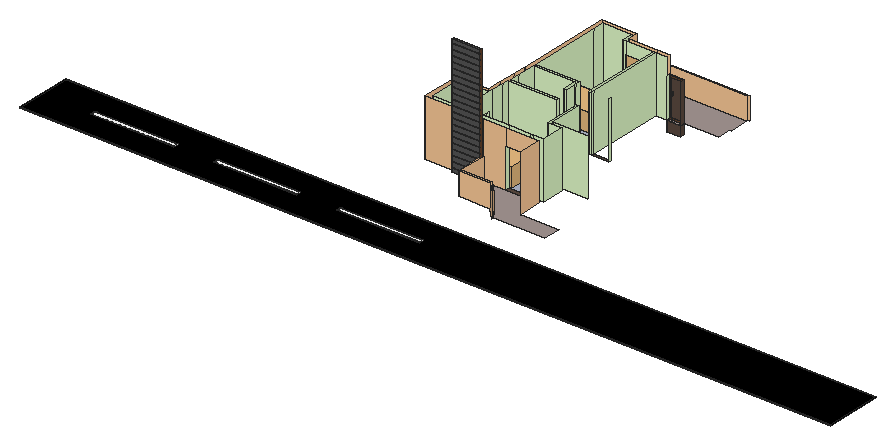
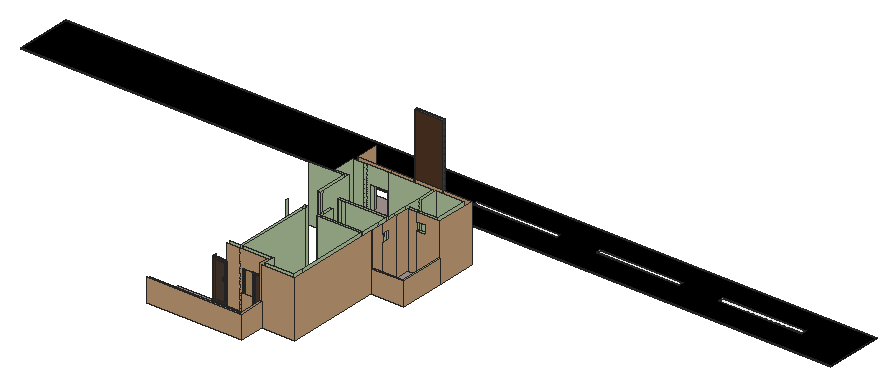
# SketchUp Ruby script. Lengths in inches.
U = 1.inch
M = Sketchup.active_model
def pt(a) = Geom::Point3d.new(a.map { |v| v * U })
def face(e, loops, mat)
  f = e.add_face(loops[0].map { |a| pt(a) })
  loops[1..].each { |l| e.add_face(l.map { |a| pt(a) }).erase! }
  f.material = f.back_material = mat if mat
  f
end
# faces: each face lists its corners as indices into pts; further lists are holes
def faces(e, pts, list, mat = nil) = list.each { |f| face(e, (f[0].is_a?(Array) ? f : [f]).map { |l| l.map { |i| pts[i] } }, mat) }
# xy, xz, yz: faces in a plane at the given z, y or x. An outline is a flat list of corners, or four numbers for a rectangle; further outlines are holes
def ring(l) = l.size == 4 ? [[l[0], l[1]], [l[2], l[1]], [l[2], l[3]], [l[0], l[3]]] : l.each_slice(2).to_a
def flat(e, list, mat, &to3) = list.each { |f| face(e, (f[0].is_a?(Array) ? f : [f]).map { |l| ring(l).map { |u, v| to3.(u, v) } }, mat) }
def xy(e, z, list, mat = nil) = flat(e, list, mat) { |x, y| [x, y, z] }
def xz(e, y, list, mat = nil) = flat(e, list, mat) { |x, z| [x, y, z] }
def yz(e, x, list, mat = nil) = flat(e, list, mat) { |y, z| [x, y, z] }
def lines(e, pts, list) = list.each { |a, b| e.add_line(pt(pts[a]), pt(pts[b])) }
# prism: a flat outline (further loops are holes) pulled along v
def prism(e, loops, v, mat = nil)
  f = face(e, loops, mat); d = Geom::Vector3d.new(v.map { |x| x * U })
  f.pushpull(f.normal.samedirection?(d) ? d.length : -d.length)
end
def box(e, o, s, mat = nil) = prism(e, [[o, [o[0] + s[0], o[1], o[2]], [o[0] + s[0], o[1] + s[1], o[2]], [o[0], o[1] + s[1], o[2]]]], [0, 0, s[2]], mat)
def at(x, y, z, deg = 0) = Geom::Transformation.translation(pt([x, y, z])) * Geom::Transformation.rotation(ORIGIN, Z_AXIS, deg.degrees)
def axes(o, x, y, z) = Geom::Transformation.new([*x, 0, *y, 0, *z, 0, *pt(o).to_a, 1])
def part(name) = M.definitions.add(name)
# library, detail: a bought-in or finely detailed component or shape, given as its bounding box
def library(name, o, s) = part(name).tap { |d| box(d.entities, o, s) }
def detail(e, o, s) = box(e.add_group.entities, o, s)
def put(e, d, t, mat = nil) = e.add_instance(d, t).tap { |i| i.material = mat if mat }
def group(e, t, mat = nil) = e.add_group.tap { |g| g.transformation = t; g.material = mat if mat }.entities
root = M.entities
M.materials.add("C02_Golden_Beige").color = [255, 205, 155]
M.materials.add("F01_Seafoam_Drift").color = [229, 255, 204]
M.materials.add("M00_Soft_Cloud").color = [255, 255, 255]
M.materials.add("M01_Silver_Fog").color = [224, 224, 224]
M.materials.add("M03_Pewter_Shine").color = [168, 168, 168]
M.materials.add("M04_Stone_Frost").color = [142, 142, 142]
M.materials.add("M06_Steel_Smoke").color = [86, 86, 86]
M.materials.add("M09_Shadow_Night").color = [0, 0, 0]
M.materials.add("Marble_03_1K").color = [175, 182, 201]
M.materials.add("Marble_06_1K").color = [165, 150, 147]
M.materials.add("Marble_20_1K").color = [172, 173, 182]
M.materials.add("Metal_06_1K").color = [238, 236, 231]
M.materials.add("Wood_Floor_12_1K").color = [92, 75, 65]
M.materials.add("Wood_Veneer_15_1K").color = [103, 69, 45]
c1 = part("Group\#73")
box(c1.entities,[0,0,0],[176.75,20.5625,0.9])
c2 = library("Toilet 005",[-7.26,-21.97,0],[14.52,21.97,16.93])
c3 = library("Marcel Lift Bed Queen",[-31.83,-34.39,0],[63.66,83.19,38.98])
c4 = part("Group\#9")
xy(c4.entities,0,[[0,0,40.3125,19.1]])
xy(c4.entities,16,[[8.1875,0.77,29.4,18.21]])
xy(c4.entities,21.0625,[[0,0,40.3125,19.1]])
xy(c4.entities,25,[[[0,0,40.3125,19.1],[8.1875,0.77,29.4,18.21]]])
xy(c4.entities,25.5,[[[0,0,40.3125,19.1],[8.1875,0.77,29.4,18.21]]],"M09_Shadow_Night")
xz(c4.entities,-0.1875,[[20.17,22.3,20.39,22.33,20.61,22.42,20.79,22.56,20.93,22.74,21.01,22.95,21.04,23.18,21.01,23.4,20.93,23.61,20.79,23.8,20.61,23.93,20.39,24.02,20.17,24.05,19.94,24.02,19.73,23.93,19.55,23.8,19.41,23.61,19.32,23.4,19.29,23.18,19.32,22.95,19.41,22.74,19.55,22.56,19.73,22.42,19.94,22.33]],"M03_Pewter_Shine")
xz(c4.entities,0,[[19.56,0,20.76,21.0625],[0,25,40.3125,25.5]],"M09_Shadow_Night")
xz(c4.entities,0,[[0,0,19.56,21.0625],[20.76,0,40.3125,21.0625],[[0,21.0625,40.3125,25],[20.17,22.3,19.94,22.33,19.73,22.42,19.55,22.56,19.41,22.74,19.32,22.95,19.29,23.18,19.32,23.4,19.41,23.61,19.55,23.8,19.73,23.93,19.94,24.02,20.17,24.05,20.39,24.02,20.61,23.93,20.79,23.8,20.93,23.61,21.01,23.4,21.04,23.18,21.01,22.95,20.93,22.74,20.79,22.56,20.61,22.42,20.39,22.33]]],"Wood_Veneer_15_1K")
xz(c4.entities,0.77,[[8.1875,16,29.4,25]])
xz(c4.entities,0.77,[[8.1875,25,29.4,25.5]],"M04_Stone_Frost")
xz(c4.entities,18.21,[[8.1875,16,29.4,25],[8.1875,25,29.4,25.5]])
xz(c4.entities,19.1,[[0,25,40.3125,25.5]],"M09_Shadow_Night")
xz(c4.entities,19.1,[[0,0,40.3125,21.0625],[0,21.0625,40.3125,25]],"Wood_Veneer_15_1K")
yz(c4.entities,0,[[0,25,19.1,25.5]],"M09_Shadow_Night")
yz(c4.entities,0,[[0,0,19.1,21.0625],[0,21.0625,19.1,25]],"Wood_Veneer_15_1K")
yz(c4.entities,8.1875,[[0.77,16,18.21,25]])
yz(c4.entities,8.1875,[[0.77,25,18.21,25.5]],"M04_Stone_Frost")
yz(c4.entities,29.4,[[0.77,16,18.21,25]])
yz(c4.entities,29.4,[[0.77,25,18.21,25.5]],"M04_Stone_Frost")
yz(c4.entities,40.3125,[[0,25,19.1,25.5]],"M09_Shadow_Night")
yz(c4.entities,40.3125,[[0,0,19.1,21.0625],[0,21.0625,19.1,25]],"Wood_Veneer_15_1K")
p = [[19.73,0,22.42],[19.94,0,22.33],[19.94,-0.1875,22.33],[19.73,-0.1875,22.42],[20.17,0,22.3],[20.17,-0.1875,22.3],
  [20.39,0,22.33],[20.39,-0.1875,22.33],[20.61,0,22.42],[20.61,-0.1875,22.42],[19.55,0,22.56],[19.55,-0.1875,22.56],
  [20.79,0,22.56],[20.79,-0.1875,22.56],[19.41,0,22.74],[19.41,-0.1875,22.74],[20.93,0,22.74],[20.93,-0.1875,22.74],
  [19.32,0,22.95],[19.32,-0.1875,22.95],[21.01,0,22.95],[21.01,-0.1875,22.95],[19.29,0,23.18],[19.29,-0.1875,23.18],
  [21.04,0,23.18],[21.04,-0.1875,23.18],[19.32,0,23.4],[19.32,-0.1875,23.4],[21.01,0,23.4],[21.01,-0.1875,23.4],
  [19.41,0,23.61],[19.41,-0.1875,23.61],[20.93,0,23.61],[20.93,-0.1875,23.61],[19.55,0,23.8],[19.55,-0.1875,23.8],
  [20.79,0,23.8],[20.79,-0.1875,23.8],[19.73,0,23.93],[19.73,-0.1875,23.93],[20.61,0,23.93],[20.61,-0.1875,23.93],
  [19.94,0,24.02],[19.94,-0.1875,24.02],[20.39,0,24.02],[20.39,-0.1875,24.02],[20.17,0,24.05],[20.17,-0.1875,24.05]]
faces(c4.entities,p,[[0,1,2,3],[1,4,5,2],[4,6,7,5],[6,8,9,7],[10,0,3,11],[8,12,13,9],[14,10,11,15],[12,16,17,13],
  [18,14,15,19],[16,20,21,17],[22,18,19,23],[20,24,25,21],[26,22,23,27],[24,28,29,25],[30,26,27,31],[28,32,33,29],
  [34,30,31,35],[32,36,37,33],[38,34,35,39],[36,40,41,37],[42,38,39,43],[40,44,45,41],[46,42,43,47],[44,46,47,45]],"M03_Pewter_Shine")
g1 = group(c4.entities,at(16.89,0,11.23),"M01_Silver_Fog")
box(g1,[0,-0.1875,0],[1.125,0.1875,4],"M03_Pewter_Shine")
g2 = group(c4.entities,at(22.02,0,11.23),"M01_Silver_Fog")
box(g2,[0,-0.1875,0],[1.125,0.1875,4],"M03_Pewter_Shine")
c5 = part("Group\#25")
xy(c5.entities,0,[[0,-3,30,0]],"Wood_Veneer_15_1K")
xy(c5.entities,3,[[3,-2.25,27,0]],"Wood_Floor_12_1K")
xy(c5.entities,3,[[3,-3,27,-2.25]],"Wood_Veneer_15_1K")
xy(c5.entities,81,[[3,-2.25,27,0]],"Wood_Floor_12_1K")
xy(c5.entities,81,[[3,-3,27,-2.25]],"Wood_Veneer_15_1K")
xy(c5.entities,84,[[0,-3,30,0]],"Wood_Veneer_15_1K")
xz(c5.entities,-3,[[[0,0,30,84],[3,3,27,81]]],"Wood_Veneer_15_1K")
xz(c5.entities,-2.25,[[3,3,27,81]],"Wood_Floor_12_1K")
xz(c5.entities,0,[[[0,0,30,84],[3,3,27,81]]],"Wood_Veneer_15_1K")
yz(c5.entities,0,[[-3,0,0,84]],"Wood_Veneer_15_1K")
yz(c5.entities,3,[[-2.25,3,0,81]],"Wood_Floor_12_1K")
yz(c5.entities,3,[[-3,3,-2.25,81]],"Wood_Veneer_15_1K")
yz(c5.entities,27,[[-2.25,3,0,81]],"Wood_Floor_12_1K")
yz(c5.entities,27,[[-3,3,-2.25,81]],"Wood_Veneer_15_1K")
yz(c5.entities,30,[[-3,0,0,84]],"Wood_Veneer_15_1K")
g3 = group(c5.entities,at(22.875,-2.25,50.47),"Metal_06_1K")
xy(g3,-5.5625,[[0,-0.48,1.25,0]],"Metal_06_1K")
xy(g3,-4.9375,[[0,-1.375,1.25,-0.48]],"Metal_06_1K")
xy(g3,-4.6875,[[0,-1.125,1.25,0]],"Metal_06_1K")
xy(g3,-4.6875,[[0,-1.375,1.25,-1.125]],"Wood_Veneer_15_1K")
xy(g3,0,[[0,-1.125,1.25,-0.5],[0,-0.5,1.25,0]],"Metal_06_1K")
xy(g3,0.25,[[0,-1.375,1.25,-1.125],[0,-1.125,1.25,-0.5]],"Metal_06_1K")
xy(g3,0.25,[[0,-0.5,1.25,0]],"Wood_Veneer_15_1K")
xy(g3,1.25,[[0,-0.5,1.25,0]],"Metal_06_1K")
xz(g3,-1.375,[[0,-4.9375,1.25,-4.6875],[0,-4.6875,1.25,0.25]],"Metal_06_1K")
xz(g3,-1.125,[[0,-4.6875,1.25,0],[0,0,1.25,0.25]],"Metal_06_1K")
xz(g3,-0.5,[[0,0.25,1.25,1.25]],"Metal_06_1K")
xz(g3,-0.5,[[0,0,1.25,0.25]],"Wood_Veneer_15_1K")
xz(g3,-0.48,[[0,-5.5625,1.25,-4.9375]],"Metal_06_1K")
xz(g3,0,[[0,0.25,1.25,1.25]],"Metal_06_1K")
xz(g3,0,[[0,-5.5625,1.25,-4.6875],[0,0,1.25,0.25]],"Wood_Veneer_15_1K")
yz(g3,0,[[-0.48,-5.5625,-0.48,-4.9375,-1.375,-4.9375,-1.375,-4.6875,0,-4.6875,0,-5.5625],[-1.375,-4.6875,-1.125,0.25],[-1.125,0,-0.5,0.25],[-0.5,0,0,0.25],[-0.5,0.25,0,1.25]],"Metal_06_1K")
yz(g3,1.25,[[-0.48,-5.5625,0,-5.5625,0,-4.6875,-1.375,-4.6875,-1.375,-4.9375,-0.48,-4.9375],[-1.375,-4.6875,-1.125,0.25],[-1.125,0,-0.5,0.25],[-0.5,0,0,0.25],[-0.5,0.25,0,1.25]],"Metal_06_1K")
c6 = library("Group\#19",[0,0,0],[54,1.88,94.04])
box(root,[1542.8125,897.17,20.5625],[9,18.21,0.4375],"Wood_Floor_12_1K")
xy(root,-0.6875,[[1705.83,1117.375,1735.83,1126.375]],"Wood_Floor_12_1K")
xy(root,11.375,[[1619.1875,1117.375,1649.1875,1126.375]],"F01_Seafoam_Drift")
xy(root,22,[[1548.8125,772.375,1689.8125,889.375],[1689.8125,772.375,1719.8125,819.6875],[1645.8125,951.6875,1677.8125,951.6875,1677.8125,1117.375,1551.8125,1117.375,1551.8125,961.375,1645.8125,961.375]],"Marble_03_1K")
xy(root,22,[[1688.52,678.6875,1797.92,678.6875,1797.92,714.6875,1716.8125,714.6875,1716.8125,763.375,1599.1,763.375,1599.1,703.375,1664.03,703.375],[1482.8125,772.375,1542.8125,841.375],[1477.8125,847.375,1542.8125,941.875],[1551.8125,1117.375,1613.1875,1141.375],[1705.83,1117.375,1735.83,1126.375],
  [1619.1875,1126.375,1809.8125,1126.375,1809.8125,1156.375,1812.8125,1156.375,1812.8125,1198.375,1619.1875,1198.375]],"Marble_06_1K")
xy(root,22,[[1551.8125,895.375,1639.8125,955.375]],"Marble_20_1K")
xy(root,22,[[1645.59,763.375,1681.59,772.375],[1542.8125,811.375,1548.8125,841.375],[1653.8125,889.375,1689.8125,895.375],[1639.8125,895.375,1645.8125,925.375],[1645.8125,945.6875,1677.8125,951.6875],
  [1683.8125,945.6875,1719.8125,951.6875],[1649.1875,1117.375,1651.0625,1126.375]],"Wood_Floor_12_1K")
xz(root,700.375,[[1596.1,21,1662.78,70]],"C02_Golden_Beige")
xz(root,703.375,[[1599.1,22,1664.03,70]],"C02_Golden_Beige")
xz(root,763.375,[[1473.8125,21,1596.1,142],[1599.1,22,1645.59,142],[1681.59,22,1716.8125,22,1716.8125,142,1645.59,142,1645.59,106,1681.59,106]],"C02_Golden_Beige")
xz(root,772.375,[[1482.8125,22,1542.8125,142],[1548.8125,22,1645.59,142],[1681.59,22,1681.59,106,1645.59,106,1645.59,142,1689.8125,142,1689.8125,22],[1689.8125,22,1695.8125,142],[1695.8125,22,1719.8125,142]],"F01_Seafoam_Drift")
xz(root,811.375,[[1542.8125,22,1548.8125,106]],"F01_Seafoam_Drift")
xz(root,819.6875,[[1689.8125,22,1719.8125,142]],"F01_Seafoam_Drift")
xz(root,825.6875,[[1695.8125,22,1770.625,142]],"F01_Seafoam_Drift")
xz(root,841.375,[[1482.8125,22,1523.47,22,1523.47,106,1504.12,106,1504.12,124,1523.47,124,1523.47,142,1482.8125,142],[1523.47,22,1542.8125,142],[1542.8125,22,1548.8125,106]],"F01_Seafoam_Drift")
xz(root,847.375,[[1477.8125,22,1477.8125,142,1523.47,142,1523.47,124,1504.12,124,1504.12,106,1523.47,106,1523.47,22],[1523.47,22,1542.8125,142]],"C02_Golden_Beige")
xz(root,889.375,[[1548.8125,22,1653.8125,142]],"F01_Seafoam_Drift")
xz(root,895.375,[[1551.8125,22,1639.8125,142],[1639.8125,22,1645.8125,142],[1645.8125,22,1653.8125,142],[1689.8125,22,1695.8125,142]],"F01_Seafoam_Drift")
xz(root,925.375,[[1639.8125,22,1645.8125,142]],"F01_Seafoam_Drift")
xz(root,941.875,[[1477.8125,22,1542.8125,70]],"C02_Golden_Beige")
xz(root,944.875,[[1473.8125,21,1542.8125,70]],"C02_Golden_Beige")
xz(root,945.6875,[[1677.8125,22,1683.8125,142]],"F01_Seafoam_Drift")
xz(root,955.375,[[1551.8125,22,1639.8125,142]],"F01_Seafoam_Drift")
xz(root,961.375,[[1551.8125,22,1645.8125,142]],"F01_Seafoam_Drift")
xz(root,1117.375,[[1619.1875,11.375,1649.1875,22],[1613.1875,22,1619.1875,142],[1673.1875,22,1677.8125,22,1677.8125,142,1619.1875,142,1619.1875,106,1673.1875,106],[1683.8125,22,1705.83,142]],"F01_Seafoam_Drift")
xz(root,1117.375,[[1705.83,-0.6875,1735.83,22],[1649.1875,22,1651.0625,106],[1651.0625,22,1673.1875,58]],"Wood_Floor_12_1K")
xz(root,1126.375,[[1673.1875,22,1673.1875,106,1619.1875,106,1619.1875,142,1677.8125,142,1677.8125,22],[1649.1875,22,1651.0625,106],[1651.0625,22,1673.1875,58],[1677.8125,22,1705.83,142]],"C02_Golden_Beige")
xz(root,1126.375,[[1619.1875,11.375,1649.1875,22]],"F01_Seafoam_Drift")
xz(root,1126.375,[[1705.83,-0.6875,1735.83,22]],"Wood_Floor_12_1K")
xz(root,1141.375,[[1551.8125,22,1613.1875,142]],"F01_Seafoam_Drift")
xz(root,1147.375,[[1542.8125,21,1613.1875,142]],"C02_Golden_Beige")
xz(root,1198.375,[[1619.1875,22,1812.8125,70]],"C02_Golden_Beige")
xz(root,1201.375,[[1613.1875,21,1815.8125,70]],"C02_Golden_Beige")
yz(root,1473.8125,[[763.375,21,847.375,142],[847.375,21,944.875,70]],"C02_Golden_Beige")
yz(root,1477.8125,[[847.375,22,941.875,70]],"F01_Seafoam_Drift")
yz(root,1482.8125,[[772.375,22,841.375,142]],"F01_Seafoam_Drift")
yz(root,1542.8125,[[944.875,21,1147.375,142],[847.375,22,877.375,142],[877.375,22,877.375,142,915.375,142,915.375,124,897.17,124,897.17,106,915.375,106,915.375,22],[915.375,22,941.875,142]],"C02_Golden_Beige")
yz(root,1542.8125,[[772.375,22,811.375,142]],"F01_Seafoam_Drift")
yz(root,1548.8125,[[772.375,22,811.375,142],[841.375,22,847.375,22,847.375,142,811.375,142,811.375,106,841.375,106],[847.375,22,877.375,142],[877.375,22,889.375,142]],"F01_Seafoam_Drift")
yz(root,1551.8125,[[895.375,22,915.375,22,915.375,106,897.17,106,897.17,124,915.375,124,915.375,142,895.375,142],[915.375,22,955.375,142],[961.375,22,1117.375,142],[1117.375,22,1141.375,142]],"F01_Seafoam_Drift")
yz(root,1596.1,[[700.375,21,763.375,70]],"C02_Golden_Beige")
yz(root,1599.1,[[703.375,22,763.375,70]],"C02_Golden_Beige")
yz(root,1613.1875,[[1147.375,21,1201.375,70]],"C02_Golden_Beige")
yz(root,1613.1875,[[1117.375,22,1141.375,142]],"F01_Seafoam_Drift")
yz(root,1619.1875,[[1126.375,22,1147.375,142],[1147.375,22,1198.375,70]],"C02_Golden_Beige")
yz(root,1619.1875,[[1117.375,11.375,1126.375,106]],"F01_Seafoam_Drift")
yz(root,1639.8125,[[925.375,22,955.375,142]],"F01_Seafoam_Drift")
yz(root,1645.59,[[763.375,22,772.375,106]],"F01_Seafoam_Drift")
yz(root,1645.8125,[[925.375,22,945.6875,142],[945.6875,22,951.6875,142],[951.6875,22,961.375,142]],"F01_Seafoam_Drift")
yz(root,1649.1875,[[1117.375,11.375,1126.375,22]],"F01_Seafoam_Drift")
yz(root,1649.1875,[[1117.375,22,1126.375,106]],"Wood_Floor_12_1K")
yz(root,1651.0625,[[1117.375,22,1126.375,58]],"Wood_Floor_12_1K")
yz(root,1653.8125,[[889.375,22,895.375,142]],"F01_Seafoam_Drift")
yz(root,1677.8125,[[945.6875,22,951.6875,142],[951.6875,22,1117.375,142]],"F01_Seafoam_Drift")
yz(root,1681.59,[[763.375,22,772.375,106]],"F01_Seafoam_Drift")
yz(root,1683.8125,[[945.6875,22,951.6875,142],[951.6875,22,1117.375,142]],"F01_Seafoam_Drift")
yz(root,1689.8125,[[819.6875,22,889.375,142],[889.375,22,895.375,142]],"F01_Seafoam_Drift")
yz(root,1695.8125,[[825.6875,22,895.375,142]],"F01_Seafoam_Drift")
yz(root,1705.83,[[1117.375,22,1126.375,106]],"F01_Seafoam_Drift")
yz(root,1705.83,[[1117.375,-0.6875,1126.375,22]],"Wood_Floor_12_1K")
yz(root,1716.8125,[[714.6875,22,763.375,142]],"C02_Golden_Beige")
yz(root,1719.8125,[[772.375,22,819.6875,142],[945.6875,22,951.6875,142]],"F01_Seafoam_Drift")
yz(root,1735.83,[[1117.375,-0.6875,1126.375,22],[1117.375,22,1126.375,106]],"Wood_Floor_12_1K")
p = [[1662.78,700.375,21],[1687.27,675.6875,21],[1687.27,675.6875,70],[1662.78,700.375,70],[1688.52,678.6875,22],[1664.03,703.375,22],
  [1664.03,703.375,70],[1688.52,678.6875,70],[1735.83,1117.375,21],[1735.83,1126.375,21],[1711.83,1117.375,21],[1711.83,1126.375,21]]
faces(root,p,[[0,1,2,3],[4,5,6,7]],"C02_Golden_Beige")
lines(root,p,[[8,9],[8,10],[11,9],[11,10]])
put(root,c1,axes([921.69,563.94,1],[1,0,0],[0,0.43638,0],[0,0,1]),"M00_Soft_Cloud")
put(root,c1,axes([1183.63,563.94,1],[1,0,0],[0,0.43638,0],[0,0,1]),"M00_Soft_Cloud")
put(root,c2,at(1483.51,804.98,22,90),"M01_Silver_Fog")
put(root,c1,axes([1445.57,563.94,1],[1,0,0],[0,0.43638,0],[0,0,1]),"M00_Soft_Cloud")
put(root,c2,at(1553.39,922.33,22,90),"M01_Silver_Fog")
g4 = group(root,at(1473.8125,763,21),"Marble_03_1K")
xy(g4,0,[[62.46,-5.8125,62.4375,0.1875,122.28,0.37,122.3,-5.63]],"Wood_Veneer_15_1K")
xy(g4,254,[[62.46,-5.8125,122.3,-5.63,122.28,0.37,62.4375,0.1875]],"M06_Steel_Smoke")
p = [[62.4375,0.1875,254],[62.4375,0.1875,0],[62.46,-5.8125,0],[62.46,-5.8125,7.89],[62.46,-5.8125,9.48],[62.46,-5.8125,19.79],
  [62.46,-5.8125,21.38],[62.46,-5.8125,31.68],[62.46,-5.8125,33.28],[62.46,-5.8125,43.57],[62.46,-5.8125,45.18],[62.46,-5.8125,55.46],
  [62.46,-5.8125,57.08],[62.46,-5.8125,67.36],[62.46,-5.8125,68.98],[62.46,-5.8125,79.25],[62.46,-5.8125,80.89],[62.46,-5.8125,91.14],
  [62.46,-5.8125,92.79],[62.46,-5.8125,103.03],[62.46,-5.8125,104.6875],[62.46,-5.8125,114.93],[62.46,-5.8125,116.59],[62.46,-5.8125,126.82],
  [62.46,-5.8125,128.49],[62.46,-5.8125,138.71],[62.46,-5.8125,140.39],[62.46,-5.8125,150.6],[62.46,-5.8125,152.29],[62.46,-5.8125,162.5],
  [62.46,-5.8125,164.19],[62.46,-5.8125,174.39],[62.46,-5.8125,176.09],[62.46,-5.8125,186.28],[62.46,-5.8125,187.99],[62.46,-5.8125,198.17],
  [62.46,-5.8125,199.89],[62.46,-5.8125,210.07],[62.46,-5.8125,211.79],[62.46,-5.8125,221.96],[62.46,-5.8125,223.69],[62.46,-5.8125,233.85],
  [62.46,-5.8125,235.6],[62.46,-5.8125,245.74],[62.46,-5.8125,247.5],[62.46,-5.8125,254],[122.3,-5.63,0],[122.3,-5.63,254],
  [122.28,0.37,0],[122.28,0.37,254],[122.28,-5.8125,247.5],[122.28,-5.8125,235.6],[122.28,-5.8125,223.69],[122.28,-5.8125,211.79],
  [122.28,-5.8125,199.89],[122.28,-5.8125,187.99],[122.28,-5.8125,176.09],[122.28,-5.8125,164.19],[122.28,-5.8125,152.29],[122.28,-5.8125,140.39],
  [122.28,-5.8125,128.49],[122.28,-5.8125,116.59],[122.28,-5.8125,104.6875],[122.28,-5.8125,92.79],[122.28,-5.8125,80.89],[122.28,-5.8125,68.98],
  [122.28,-5.8125,57.08],[122.28,-5.8125,45.18],[122.28,-5.8125,33.28],[122.28,-5.8125,21.38],[122.28,-5.8125,9.48],[122.28,-5.8125,245.74],
  [122.28,-5.8125,233.85],[122.28,-5.8125,221.96],[122.28,-5.8125,210.07],[122.28,-5.8125,198.17],[122.28,-5.8125,186.28],[122.28,-5.8125,174.39],
  [122.28,-5.8125,162.5],[122.28,-5.8125,150.6],[122.28,-5.8125,138.71],[122.28,-5.8125,126.82],[122.28,-5.8125,114.93],[122.28,-5.8125,103.03],
  [122.28,-5.8125,91.14],[122.28,-5.8125,79.25],[122.28,-5.8125,67.36],[122.28,-5.8125,55.46],[122.28,-5.8125,43.57],[122.28,-5.8125,31.68],
  [122.28,-5.8125,19.79],[122.28,-5.8125,7.89]]
faces(g4,p,[[0,1,2,3,4,5,6,7,8,9,10,11,12,13,14,15,16,17,18,19,20,21,22,23,24,25,26,27,28,29,30,31,32,33,34,35,36,37,38,39,40,41,42,43,44,45],[3,2,46,47,45,44,43,42,41,40,39,38,37,36,35,34,33,32,31,30,29,28,27,26,25,24,23,22,21,20,19,18,17,16,15,14,13,12,11,10,9,8,7,6,5,4]],"M06_Steel_Smoke")
faces(g4,p,[[48,49,47,46],[1,0,49,48]],"Wood_Veneer_15_1K")
lines(g4,p,[[44,50],[42,51],[40,52],[38,53],[36,54],[34,55],[32,56],[30,57],[28,58],[26,59],[24,60],[22,61],
  [20,62],[18,63],[16,64],[14,65],[12,66],[10,67],[8,68],[6,69],[4,70],[43,71],[41,72],[39,73],
  [37,74],[35,75],[33,76],[31,77],[29,78],[27,79],[25,80],[23,81],[21,82],[19,83],[17,84],[15,85],
  [13,86],[11,87],[9,88],[7,89],[5,90],[3,91]])
put(root,c3,at(1603.75,1033.625,22,90),"M00_Soft_Cloud")
put(root,c3,at(1616.68,826.18,22,180),"M00_Soft_Cloud")
put(root,c4,at(1599.5,936.27,22),"M00_Soft_Cloud")
put(root,c5,at(1649.1875,1123.375,22,-180),"M00_Soft_Cloud")
put(root,c6,at(1619.1875,1116.34,22),"M00_Soft_Cloud")
g5 = group(root,at(1284.6,522.9375,0))
box(g5,[-469.17,-14.92,0],[1727.99,121.48,1],"M09_Shadow_Night")
put(root,c5,at(1735.83,1123.375,22,-180),"M00_Soft_Cloud")
